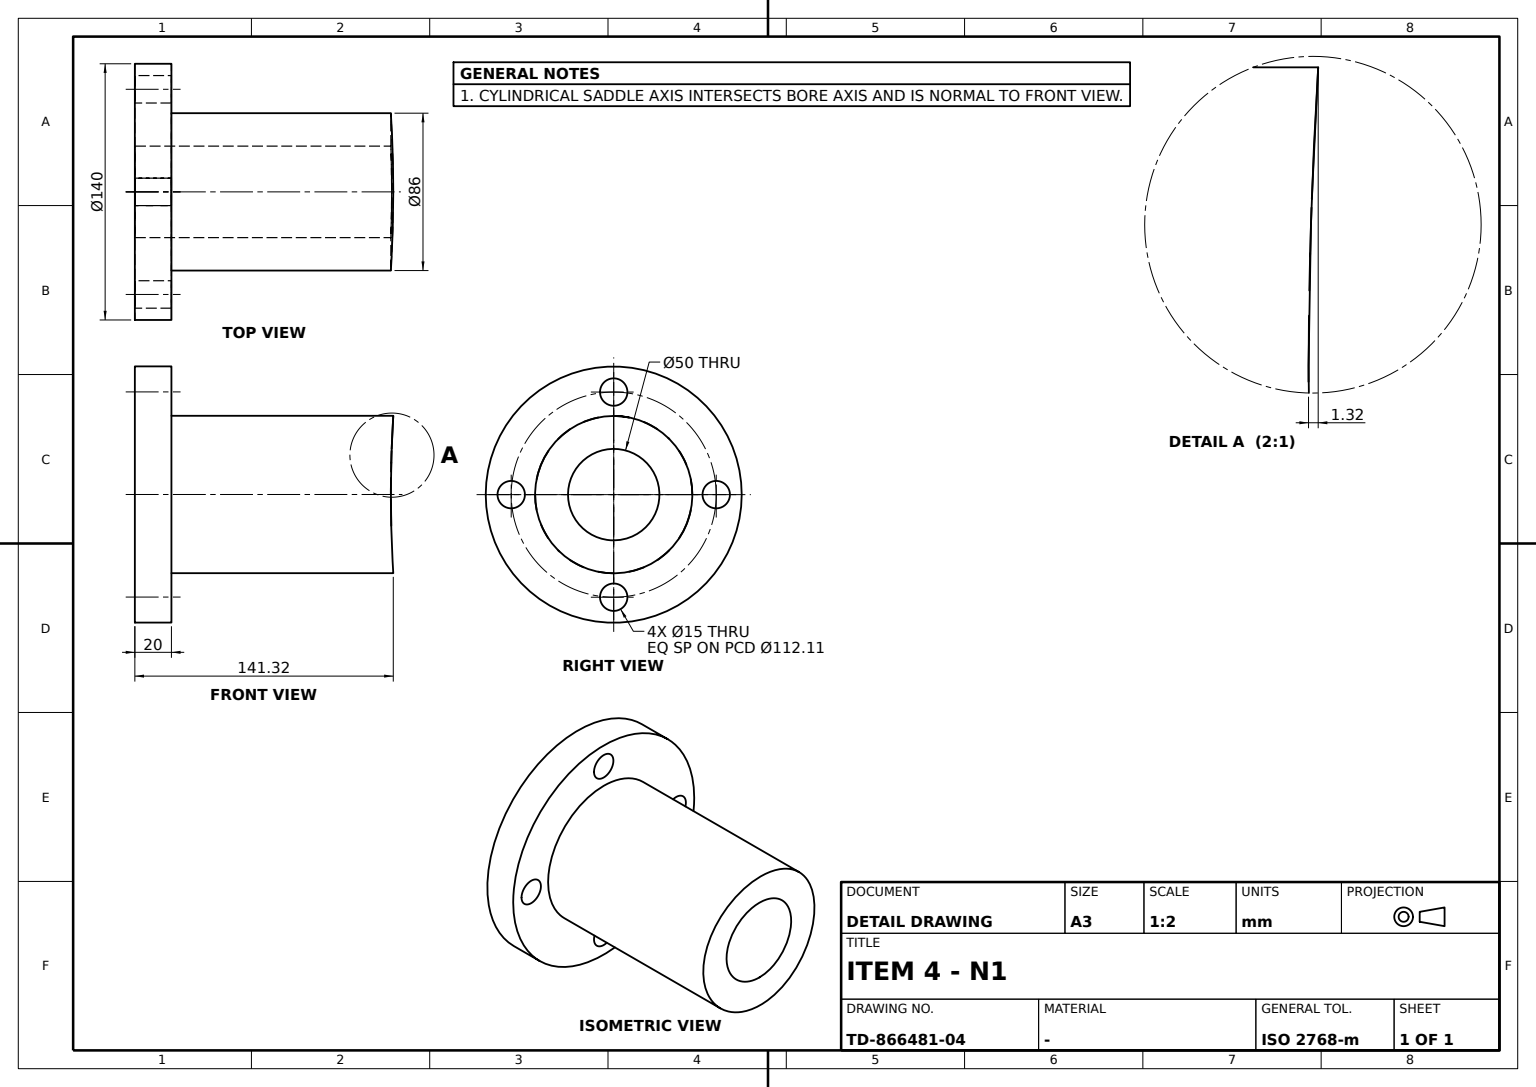
ISO-10303-21;
HEADER;
FILE_DESCRIPTION((''),'2;1');
FILE_NAME('','',(''),(''),'','','');
FILE_SCHEMA(('AUTOMOTIVE_DESIGN'));
ENDSEC;
DATA;
#1=APPLICATION_CONTEXT('');
#2=PRODUCT_CONTEXT('',#1,'mechanical');
#3=PRODUCT('','','',(#2));
#4=PRODUCT_DEFINITION_FORMATION('','',#3);
#5=PRODUCT_DEFINITION_CONTEXT('',#1,'design');
#6=PRODUCT_DEFINITION('','',#4,#5);
#7=PRODUCT_DEFINITION_SHAPE('','',#6);
#8=(LENGTH_UNIT()NAMED_UNIT(*)SI_UNIT(.MILLI.,.METRE.));
#9=(NAMED_UNIT(*)PLANE_ANGLE_UNIT()SI_UNIT($,.RADIAN.));
#10=(NAMED_UNIT(*)SI_UNIT($,.STERADIAN.)SOLID_ANGLE_UNIT());
#11=UNCERTAINTY_MEASURE_WITH_UNIT(LENGTH_MEASURE(0.005),#8,'distance_accuracy_value','');
#12=(GEOMETRIC_REPRESENTATION_CONTEXT(3)GLOBAL_UNCERTAINTY_ASSIGNED_CONTEXT((#11))GLOBAL_UNIT_ASSIGNED_CONTEXT((#8,#9,#10))REPRESENTATION_CONTEXT('',''));
#13=CARTESIAN_POINT('',(0.,-820.,701.443054));
#14=VERTEX_POINT('',#13);
#15=CARTESIAN_POINT('',(0.,-820.,693.943054));
#16=DIRECTION('',(0.,1.,0.));
#17=DIRECTION('',(0.,0.,1.));
#18=AXIS2_PLACEMENT_3D('',#15,#16,#17);
#19=CIRCLE('',#18,7.5);
#20=EDGE_CURVE('',#14,#14,#19,.F.);
#21=ORIENTED_EDGE('',*,*,#20,.T.);
#22=EDGE_LOOP('',(#21));
#23=FACE_BOUND('',#22,.T.);
#24=CARTESIAN_POINT('',(0.,-820.,820.));
#25=VERTEX_POINT('',#24);
#26=CARTESIAN_POINT('',(0.,-820.,750.));
#27=AXIS2_PLACEMENT_3D('',#26,#16,#17);
#28=CIRCLE('',#27,70.);
#29=EDGE_CURVE('',#25,#25,#28,.F.);
#30=ORIENTED_EDGE('',*,*,#29,.F.);
#31=EDGE_LOOP('',(#30));
#32=FACE_BOUND('',#31,.T.);
#33=CARTESIAN_POINT('',(56.056946,-820.,757.5));
#34=VERTEX_POINT('',#33);
#35=CARTESIAN_POINT('',(56.056946,-820.,750.));
#36=AXIS2_PLACEMENT_3D('',#35,#16,#17);
#37=CIRCLE('',#36,7.5);
#38=EDGE_CURVE('',#34,#34,#37,.F.);
#39=ORIENTED_EDGE('',*,*,#38,.T.);
#40=EDGE_LOOP('',(#39));
#41=FACE_BOUND('',#40,.T.);
#42=CARTESIAN_POINT('',(0.,-820.,793.));
#43=VERTEX_POINT('',#42);
#44=CIRCLE('',#27,43.);
#45=EDGE_CURVE('',#43,#43,#44,.T.);
#46=ORIENTED_EDGE('',*,*,#45,.F.);
#47=EDGE_LOOP('',(#46));
#48=FACE_BOUND('',#47,.T.);
#49=CARTESIAN_POINT('',(0.,-820.,813.556946));
#50=VERTEX_POINT('',#49);
#51=CARTESIAN_POINT('',(0.,-820.,806.056946));
#52=AXIS2_PLACEMENT_3D('',#51,#16,#17);
#53=CIRCLE('',#52,7.5);
#54=EDGE_CURVE('',#50,#50,#53,.F.);
#55=ORIENTED_EDGE('',*,*,#54,.T.);
#56=EDGE_LOOP('',(#55));
#57=FACE_BOUND('',#56,.T.);
#58=CARTESIAN_POINT('',(-56.056946,-820.,757.5));
#59=VERTEX_POINT('',#58);
#60=CARTESIAN_POINT('',(-56.056946,-820.,750.));
#61=AXIS2_PLACEMENT_3D('',#60,#16,#17);
#62=CIRCLE('',#61,7.5);
#63=EDGE_CURVE('',#59,#59,#62,.F.);
#64=ORIENTED_EDGE('',*,*,#63,.T.);
#65=EDGE_LOOP('',(#64));
#66=FACE_BOUND('',#65,.T.);
#67=CARTESIAN_POINT('',(0.,-820.,0.));
#68=DIRECTION('',(-1.,0.,0.));
#69=AXIS2_PLACEMENT_3D('',#67,#16,#68);
#70=PLANE('',#69);
#71=ADVANCED_FACE('',(#23,#32,#41,#48,#57,#66),#70,.T.);
#72=CARTESIAN_POINT('',(0.,-840.,798.556946));
#73=VERTEX_POINT('',#72);
#74=CARTESIAN_POINT('',(0.,-840.,806.056946));
#75=DIRECTION('',(0.,-1.,0.));
#76=DIRECTION('',(0.,0.,-1.));
#77=AXIS2_PLACEMENT_3D('',#74,#75,#76);
#78=CIRCLE('',#77,7.5);
#79=EDGE_CURVE('',#73,#73,#78,.T.);
#80=ORIENTED_EDGE('',*,*,#79,.T.);
#81=EDGE_LOOP('',(#80));
#82=FACE_BOUND('',#81,.T.);
#83=ORIENTED_EDGE('',*,*,#54,.F.);
#84=EDGE_LOOP('',(#83));
#85=FACE_BOUND('',#84,.T.);
#86=CARTESIAN_POINT('',(0.,-830.,806.056946));
#87=DIRECTION('',(1.,0.,0.));
#88=AXIS2_PLACEMENT_3D('',#86,#75,#87);
#89=CYLINDRICAL_SURFACE('',#88,7.5);
#90=ADVANCED_FACE('',(#82,#85),#89,.F.);
#91=ORIENTED_EDGE('',*,*,#45,.T.);
#92=EDGE_LOOP('',(#91));
#93=FACE_BOUND('',#92,.T.);
#94=CARTESIAN_POINT('',(-43.,-698.678037,750.));
#95=VERTEX_POINT('',#94);
#96=CARTESIAN_POINT('',(-42.43097,-698.713376,741.47583));
#97=CARTESIAN_POINT('',(-43.279785,-698.660649,750.025972));
#98=CARTESIAN_POINT('',(-42.449888,-698.712252,758.42028));
#99=CARTESIAN_POINT('',(-39.97048,-698.860293,766.589917));
#100=CARTESIAN_POINT('',(-36.005211,-699.07868,774.010058));
#101=CARTESIAN_POINT('',(-30.588402,-699.339921,780.616285));
#102=CARTESIAN_POINT('',(-24.07131,-699.597771,785.961771));
#103=CARTESIAN_POINT('',(-16.57762,-699.818486,789.979477));
#104=CARTESIAN_POINT('',(-8.442889,-699.965467,792.442964));
#105=CARTESIAN_POINT('',(-0.047803,-700.01727,793.278595));
#106=CARTESIAN_POINT('',(8.456705,-699.96545,792.442593));
#107=CARTESIAN_POINT('',(16.510689,-699.81984,790.002301));
#108=CARTESIAN_POINT('',(24.03914,-699.599095,785.989272));
#109=CARTESIAN_POINT('',(30.576284,-699.340367,780.622272));
#110=CARTESIAN_POINT('',(35.959295,-699.081073,774.085073));
#111=CARTESIAN_POINT('',(39.97873,-698.859866,766.564388));
#112=CARTESIAN_POINT('',(42.430982,-698.713375,758.524116));
#113=CARTESIAN_POINT('',(43.279785,-698.660649,749.973957));
#114=CARTESIAN_POINT('',(42.449877,-698.712253,741.579666));
#115=CARTESIAN_POINT('',(39.970461,-698.860294,733.410038));
#116=CARTESIAN_POINT('',(36.005188,-699.078682,725.989909));
#117=CARTESIAN_POINT('',(30.588379,-699.339922,719.383693));
#118=CARTESIAN_POINT('',(24.07129,-699.597772,714.038215));
#119=CARTESIAN_POINT('',(16.577605,-699.818486,710.020517));
#120=CARTESIAN_POINT('',(8.442881,-699.965468,707.557035));
#121=CARTESIAN_POINT('',(0.047803,-700.01727,706.721405));
#122=CARTESIAN_POINT('',(-8.456697,-699.96545,707.557405));
#123=CARTESIAN_POINT('',(-16.510674,-699.81984,709.997693));
#124=CARTESIAN_POINT('',(-24.03912,-699.599095,714.010715));
#125=CARTESIAN_POINT('',(-30.57626,-699.340368,719.377705));
#126=CARTESIAN_POINT('',(-35.959273,-699.081074,725.914894));
#127=CARTESIAN_POINT('',(-39.978711,-698.859867,733.435566));
#128=B_SPLINE_CURVE_WITH_KNOTS('',3,(#96,#97,#98,#99,#100,#101,#102,#103,#104,#105,#106,#107,#108,#109,#110,#111,#112,#113,#114,#115,#116,#117,#118,#119,#120,#121,#122,#123,#124,#125,#126,#127,#96,#97,#98),.UNSPECIFIED.,.T.,.F.,(1,1,1,1,1,1,1,1,1,1,1,1,1,1,1,1,1,1,1,1,1,1,1,1,1,1,1,1,1,1,1,1,1,1,1,1,1,1,1),(-0.02520767,-0.016805114,-0.008402557,0.,0.008402557,0.016805114,0.02520767,0.033610227,0.042012784,0.050415341,0.058817897,0.067220454,0.075623011,0.084025568,0.092428124,0.100830681,0.109233238,0.117635795,0.126038351,0.134440908,0.142843465,0.151246022,0.159648578,0.168051135,0.176453692,0.184856249,0.193258805,0.201661362,0.210063919,0.218466476,0.226869032,0.235271589,0.243674146,0.252076703,0.260479259,0.268881816,0.277284373,0.28568693,0.294089486),.UNSPECIFIED.);
#129=EDGE_CURVE('',#95,#95,#128,.T.);
#130=ORIENTED_EDGE('',*,*,#129,.F.);
#131=EDGE_LOOP('',(#130));
#132=FACE_BOUND('',#131,.T.);
#133=CARTESIAN_POINT('',(0.,-59.34,750.));
#134=AXIS2_PLACEMENT_3D('',#133,#16,#68);
#135=CYLINDRICAL_SURFACE('',#134,43.);
#136=ADVANCED_FACE('',(#93,#132),#135,.T.);
#137=ORIENTED_EDGE('',*,*,#38,.F.);
#138=EDGE_LOOP('',(#137));
#139=FACE_BOUND('',#138,.T.);
#140=CARTESIAN_POINT('',(56.056946,-840.,742.5));
#141=VERTEX_POINT('',#140);
#142=CARTESIAN_POINT('',(56.056946,-840.,750.));
#143=AXIS2_PLACEMENT_3D('',#142,#75,#76);
#144=CIRCLE('',#143,7.5);
#145=EDGE_CURVE('',#141,#141,#144,.T.);
#146=ORIENTED_EDGE('',*,*,#145,.T.);
#147=EDGE_LOOP('',(#146));
#148=FACE_BOUND('',#147,.T.);
#149=CARTESIAN_POINT('',(56.056946,-830.,750.));
#150=AXIS2_PLACEMENT_3D('',#149,#75,#87);
#151=CYLINDRICAL_SURFACE('',#150,7.5);
#152=ADVANCED_FACE('',(#139,#148),#151,.F.);
#153=ORIENTED_EDGE('',*,*,#20,.F.);
#154=EDGE_LOOP('',(#153));
#155=FACE_BOUND('',#154,.T.);
#156=CARTESIAN_POINT('',(0.,-840.,686.443054));
#157=VERTEX_POINT('',#156);
#158=CARTESIAN_POINT('',(0.,-840.,693.943054));
#159=AXIS2_PLACEMENT_3D('',#158,#75,#76);
#160=CIRCLE('',#159,7.5);
#161=EDGE_CURVE('',#157,#157,#160,.T.);
#162=ORIENTED_EDGE('',*,*,#161,.T.);
#163=EDGE_LOOP('',(#162));
#164=FACE_BOUND('',#163,.T.);
#165=CARTESIAN_POINT('',(0.,-830.,693.943054));
#166=AXIS2_PLACEMENT_3D('',#165,#75,#87);
#167=CYLINDRICAL_SURFACE('',#166,7.5);
#168=ADVANCED_FACE('',(#155,#164),#167,.F.);
#169=ORIENTED_EDGE('',*,*,#161,.F.);
#170=EDGE_LOOP('',(#169));
#171=FACE_BOUND('',#170,.T.);
#172=CARTESIAN_POINT('',(0.,-840.,680.));
#173=VERTEX_POINT('',#172);
#174=CARTESIAN_POINT('',(0.,-840.,750.));
#175=AXIS2_PLACEMENT_3D('',#174,#75,#76);
#176=CIRCLE('',#175,70.);
#177=EDGE_CURVE('',#173,#173,#176,.T.);
#178=ORIENTED_EDGE('',*,*,#177,.T.);
#179=EDGE_LOOP('',(#178));
#180=FACE_BOUND('',#179,.T.);
#181=CARTESIAN_POINT('',(0.,-840.,725.));
#182=VERTEX_POINT('',#181);
#183=CIRCLE('',#175,25.);
#184=EDGE_CURVE('',#182,#182,#183,.T.);
#185=ORIENTED_EDGE('',*,*,#184,.F.);
#186=EDGE_LOOP('',(#185));
#187=FACE_BOUND('',#186,.T.);
#188=CARTESIAN_POINT('',(-56.056946,-840.,742.5));
#189=VERTEX_POINT('',#188);
#190=CARTESIAN_POINT('',(-56.056946,-840.,750.));
#191=AXIS2_PLACEMENT_3D('',#190,#75,#76);
#192=CIRCLE('',#191,7.5);
#193=EDGE_CURVE('',#189,#189,#192,.T.);
#194=ORIENTED_EDGE('',*,*,#193,.F.);
#195=EDGE_LOOP('',(#194));
#196=FACE_BOUND('',#195,.T.);
#197=ORIENTED_EDGE('',*,*,#79,.F.);
#198=EDGE_LOOP('',(#197));
#199=FACE_BOUND('',#198,.T.);
#200=ORIENTED_EDGE('',*,*,#145,.F.);
#201=EDGE_LOOP('',(#200));
#202=FACE_BOUND('',#201,.T.);
#203=CARTESIAN_POINT('',(0.,-840.,0.));
#204=AXIS2_PLACEMENT_3D('',#203,#75,#87);
#205=PLANE('',#204);
#206=ADVANCED_FACE('',(#171,#180,#187,#196,#199,#202),#205,.T.);
#207=ORIENTED_EDGE('',*,*,#29,.T.);
#208=EDGE_LOOP('',(#207));
#209=FACE_BOUND('',#208,.T.);
#210=ORIENTED_EDGE('',*,*,#177,.F.);
#211=EDGE_LOOP('',(#210));
#212=FACE_BOUND('',#211,.T.);
#213=CARTESIAN_POINT('',(0.,-830.,750.));
#214=AXIS2_PLACEMENT_3D('',#213,#75,#87);
#215=CYLINDRICAL_SURFACE('',#214,70.);
#216=ADVANCED_FACE('',(#209,#212),#215,.T.);
#217=ORIENTED_EDGE('',*,*,#184,.T.);
#218=EDGE_LOOP('',(#217));
#219=FACE_BOUND('',#218,.T.);
#220=CARTESIAN_POINT('',(25.,-699.553429,750.));
#221=VERTEX_POINT('',#220);
#222=CARTESIAN_POINT('',(23.693387,-699.60194,759.831709));
#223=CARTESIAN_POINT('',(25.652824,-699.529191,749.997725));
#224=CARTESIAN_POINT('',(23.695316,-699.601871,740.177392));
#225=CARTESIAN_POINT('',(18.136191,-699.776784,731.862076));
#226=CARTESIAN_POINT('',(9.824044,-699.951542,726.306392));
#227=CARTESIAN_POINT('',(0.01807,-700.024108,724.350286));
#228=CARTESIAN_POINT('',(-9.794368,-699.952023,726.292499));
#229=CARTESIAN_POINT('',(-18.125305,-699.777121,731.849051));
#230=CARTESIAN_POINT('',(-23.693391,-699.60194,740.168301));
#231=CARTESIAN_POINT('',(-25.652824,-699.529191,750.002292));
#232=CARTESIAN_POINT('',(-23.695312,-699.601871,759.822617));
#233=CARTESIAN_POINT('',(-18.136185,-699.776784,768.137929));
#234=CARTESIAN_POINT('',(-9.82404,-699.951542,773.693609));
#235=CARTESIAN_POINT('',(-0.01807,-700.024108,775.649714));
#236=CARTESIAN_POINT('',(9.794365,-699.952023,773.707502));
#237=CARTESIAN_POINT('',(18.1253,-699.777121,768.150954));
#238=B_SPLINE_CURVE_WITH_KNOTS('',3,(#222,#223,#224,#225,#226,#227,#228,#229,#230,#231,#232,#233,#234,#235,#236,#237,#222,#223,#224),.UNSPECIFIED.,.T.,.F.,(1,1,1,1,1,1,1,1,1,1,1,1,1,1,1,1,1,1,1,1,1,1,1),(-0.029306791,-0.019537861,-0.00976893,0.,0.00976893,0.019537861,0.029306791,0.039075721,0.048844652,0.058613582,0.068382512,0.078151443,0.087920373,0.097689303,0.107458234,0.117227164,0.126996094,0.136765024,0.146533955,0.156302885,0.166071815,0.175840746,0.185609676),.UNSPECIFIED.);
#239=EDGE_CURVE('',#221,#221,#238,.T.);
#240=ORIENTED_EDGE('',*,*,#239,.T.);
#241=EDGE_LOOP('',(#240));
#242=FACE_BOUND('',#241,.T.);
#243=CYLINDRICAL_SURFACE('',#214,25.);
#244=ADVANCED_FACE('',(#219,#242),#243,.F.);
#245=ORIENTED_EDGE('',*,*,#193,.T.);
#246=EDGE_LOOP('',(#245));
#247=FACE_BOUND('',#246,.T.);
#248=ORIENTED_EDGE('',*,*,#63,.F.);
#249=EDGE_LOOP('',(#248));
#250=FACE_BOUND('',#249,.T.);
#251=CARTESIAN_POINT('',(-56.056946,-830.,750.));
#252=AXIS2_PLACEMENT_3D('',#251,#75,#87);
#253=CYLINDRICAL_SURFACE('',#252,7.5);
#254=ADVANCED_FACE('',(#247,#250),#253,.F.);
#255=ORIENTED_EDGE('',*,*,#129,.T.);
#256=EDGE_LOOP('',(#255));
#257=FACE_BOUND('',#256,.T.);
#258=ORIENTED_EDGE('',*,*,#239,.F.);
#259=EDGE_LOOP('',(#258));
#260=FACE_BOUND('',#259,.T.);
#261=CARTESIAN_POINT('',(0.,0.,860.));
#262=AXIS2_PLACEMENT_3D('',#261,#17,#87);
#263=CYLINDRICAL_SURFACE('',#262,700.);
#264=ADVANCED_FACE('',(#257,#260),#263,.F.);
#265=CLOSED_SHELL('',(#71,#90,#136,#152,#168,#206,#216,#244,#254,#264));
#266=MANIFOLD_SOLID_BREP('',#265);
#267=ADVANCED_BREP_SHAPE_REPRESENTATION('',(#266),#12);
#268=SHAPE_DEFINITION_REPRESENTATION(#7,#267);
ENDSEC;
END-ISO-10303-21;
